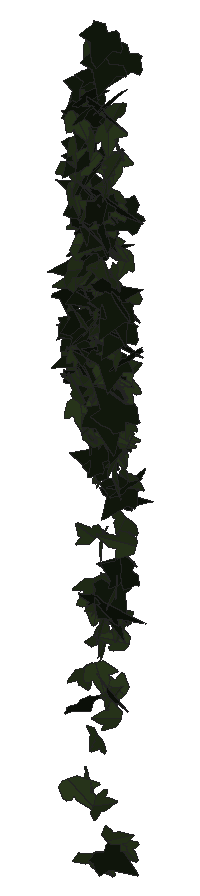
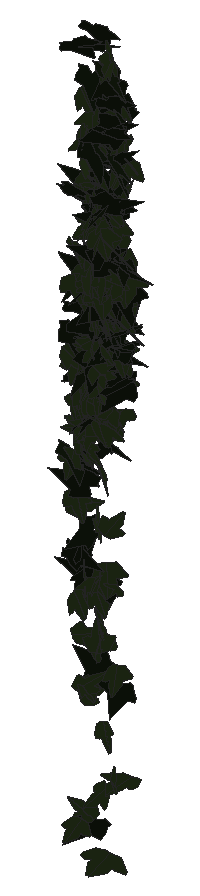
# SketchUp Ruby script. Lengths in millimetres.
U = 1.mm
M = Sketchup.active_model
def pt(a) = Geom::Point3d.new(a.map { |v| v * U })
def face(e, loops, mat)
  f = e.add_face(loops[0].map { |a| pt(a) })
  loops[1..].each { |l| e.add_face(l.map { |a| pt(a) }).erase! }
  f.material = f.back_material = mat if mat
  f
end
# faces: each face lists its corners as indices into pts; further lists are holes
def faces(e, pts, list, mat = nil) = list.each { |f| face(e, (f[0].is_a?(Array) ? f : [f]).map { |l| l.map { |i| pts[i] } }, mat) }
# xy, xz, yz: faces in a plane at the given z, y or x. An outline is a flat list of corners, or four numbers for a rectangle; further outlines are holes
def ring(l) = l.size == 4 ? [[l[0], l[1]], [l[2], l[1]], [l[2], l[3]], [l[0], l[3]]] : l.each_slice(2).to_a
def flat(e, list, mat, &to3) = list.each { |f| face(e, (f[0].is_a?(Array) ? f : [f]).map { |l| ring(l).map { |u, v| to3.(u, v) } }, mat) }
def xy(e, z, list, mat = nil) = flat(e, list, mat) { |x, y| [x, y, z] }
def xz(e, y, list, mat = nil) = flat(e, list, mat) { |x, z| [x, y, z] }
def yz(e, x, list, mat = nil) = flat(e, list, mat) { |y, z| [x, y, z] }
def lines(e, pts, list) = list.each { |a, b| e.add_line(pt(pts[a]), pt(pts[b])) }
# prism: a flat outline (further loops are holes) pulled along v
def prism(e, loops, v, mat = nil)
  f = face(e, loops, mat); d = Geom::Vector3d.new(v.map { |x| x * U })
  f.pushpull(f.normal.samedirection?(d) ? d.length : -d.length)
end
def box(e, o, s, mat = nil) = prism(e, [[o, [o[0] + s[0], o[1], o[2]], [o[0] + s[0], o[1] + s[1], o[2]], [o[0], o[1] + s[1], o[2]]]], [0, 0, s[2]], mat)
def at(x, y, z, deg = 0) = Geom::Transformation.translation(pt([x, y, z])) * Geom::Transformation.rotation(ORIGIN, Z_AXIS, deg.degrees)
def axes(o, x, y, z) = Geom::Transformation.new([*x, 0, *y, 0, *z, 0, *pt(o).to_a, 1])
def part(name) = M.definitions.add(name)
# library, detail: a bought-in or finely detailed component or shape, given as its bounding box
def library(name, o, s) = part(name).tap { |d| box(d.entities, o, s) }
def detail(e, o, s) = box(e.add_group.entities, o, s)
def put(e, d, t, mat = nil) = e.add_instance(d, t).tap { |i| i.material = mat if mat }
def group(e, t, mat = nil) = e.add_group.tap { |g| g.transformation = t; g.material = mat if mat }.entities
root = M.entities
M.materials.add("efeu1").color = [18, 25, 13]
M.materials.add("efeu2").color = [43, 57, 29]
c1 = part("ivyleaf_10")
p = [[0,12.8,-0.8],[-1.5,51.3,-10.9],[-4.9,51,-11.6],[-13.6,26.5,-7.3],[-13.2,15.9,-4.6],[-21.1,19.3,-7.2],
  [-29.5,16.3,-8.3],[-29.2,8.3,-6.2],[-19.7,-9.8,0.5],[-7.6,-13,4],[1,-12.2,5.8],[-0.4,51.1,-11.1],
  [-1.5,51.1,-10.9],[1,-12.4,5.9],[16.9,-12.4,3.5],[35.1,9.1,-5.1],[35,12.9,-6.1],[20.5,16.4,-4.9],
  [15.8,15,-3.8],[15.3,27.6,-7.1],[12.8,31.3,-7.8]]
faces(c1.entities,p,[[0,1,2,3,4,5,6,7,8,9,10],[11,12,0,13,14,15,16,17,18,19,20]],"efeu2")
c2 = part("ivyleaf_9")
p = [[39.1,54.8,31.7],[34.5,51.8,30.2],[-5.3,25.2,17.3],[-17.9,28.3,20.9],[-21.6,21.7,17],[-20.2,4.3,5.3],
  [-22.9,-0.3,2.5],[-17.1,-4,-0.6],[-2,-2.1,-1.2],[-0.7,-15.4,-10.1],[16.6,-22.3,-16.7],[21.1,-15.1,-12.5],
  [32.7,-10.7,-11],[46.1,-1.8,-6.6],[30.8,11.2,3.8]]
faces(c2.entities,p,[[0,1,2,3,4,5,6,7,8,9,10,11,12,13,14]],"efeu1")
put(root,c1,axes([752.7,985.2,1113.9],[-0.74272,0.32931,-0.52967],[-0.59636,0.20777,0.69102],[0.47258,0.77975,0.03957]))
put(root,c2,axes([734.6,998.7,1013.6],[0.71888,0.48535,0.05808],[0.0471,0.04448,-0.76333],[-0.59448,0.59043,0.00976]))
put(root,c1,axes([746.1,992.7,1011.5],[-0.86277,0.0268,-0.17998],[-0.21923,0.01065,0.70769],[0.03488,0.72965,-0.00372]))
put(root,c2,axes([744.8,980.7,1167.3],[0.45026,0.58354,-0.42423],[-0.26636,-0.36384,-0.6904],[-0.8389,0.42872,-0.00848]))
put(root,c2,axes([734.3,1024.5,1017.5],[-0.16118,-0.77907,-0.00625],[-0.00493,0.00702,-0.79017],[0.95048,-0.13207,-0.00516]))
put(root,c1,axes([743.7,985.2,1184.5],[-0.71292,-0.63034,0.00049],[0.00698,-0.00597,-0.8595],[0.76898,-0.58433,0.00825]))
put(root,c2,axes([758.7,1001.5,1208.6],[-0.84853,0.10376,0.4092],[-0.50488,-0.01181,-0.70039],[-0.10172,-0.80687,0.06287]))
put(root,c1,axes([744,999.7,1067.4],[-0.31665,-0.79481,0.09066],[-0.01002,-0.09266,-0.83586],[0.97591,-0.25884,0.02083]))
put(root,c2,axes([746.7,1016.1,1408.8],[-0.72738,0.31029,-0.35451],[0.33499,-0.23579,-0.66816],[-0.46706,-0.65234,0.07288]))
put(root,c1,axes([739,983.2,1341.1],[-0.18555,0.78695,0.1091],[-0.04414,0.1041,-0.80136],[-0.96826,-0.15555,0.01563]))
put(root,c2,axes([758.8,1017.5,1320.6],[-0.28431,0.09191,0.72797],[-0.89505,-0.01646,-0.23278],[-0.01491,-0.76418,0.09257]))
put(root,c1,axes([736,1006.1,962.2],[0.62964,0.64605,0.08333],[0.08075,0.05376,-0.82669],[-0.7906,0.52001,-0.01807]))
put(root,c2,axes([747.1,1019.8,1506.6],[-0.82677,-0.409,-0.01842],[0.01997,0.00852,-0.79154],[0.49909,-0.67788,0.00117]))
put(root,c2,axes([744.2,1009.6,1401.8],[-0.48567,-0.60806,0.27911],[-0.17746,-0.23836,-0.72674],[0.79673,-0.42375,0.00827]))
put(root,c2,axes([751.5,981.2,1221.1],[-0.06903,0.74396,0.27596],[-0.04233,0.27407,-0.746],[-0.96714,-0.06509,0.01296]))
put(root,c2,axes([740.4,1014.4,1457.2],[-0.32635,-0.71367,0.01173],[-0.00513,-0.01096,-0.76215],[0.87078,-0.26753,-0.00009]))
put(root,c2,axes([756.5,1008.3,1060.5],[-0.84556,-0.25006,0.34141],[-0.37588,-0.15097,-0.73603],[0.35394,-0.75772,0.03397]))
put(root,c1,axes([742.2,988.9,1421.9],[0.10068,0.76939,-0.10646],[-0.03631,-0.10384,-0.77358],[-0.9469,0.08579,0.01835]))
put(root,c2,axes([733.9,998.7,1103],[0.03434,-0.77163,-0.17513],[0.21582,0.17695,-0.75118],[0.9409,-0.01242,0.1787]))
put(root,c1,axes([757.1,979.1,994.5],[-0.50932,0.34946,-0.48835],[-0.47788,0.29235,0.54405],[0.5553,0.57211,0.02028]))
put(root,c1,axes([737.1,1002.6,1493.3],[0.76919,-0.31526,0.33383],[0.36271,-0.15187,-0.70491],[0.42691,0.69706,-0.00259]))
put(root,c1,axes([744.1,973.6,1211.4],[-0.12272,-0.31156,-0.81234],[0.23913,0.78861,-0.32673],[1.03416,-0.21932,-0.02084]))
put(root,c1,axes([746.2,1003,509.9],[-0.32891,-0.6822,-0.18443],[0.14876,0.14953,-0.73134],[0.84923,-0.29041,0.05668]))
put(root,c1,axes([745.1,995.2,1064.3],[0.38522,0.78872,-0.0383],[-0.15994,0.01168,-0.84019],[-0.95,0.31786,0.12592]))
put(root,c1,axes([743.1,983.6,1382.8],[-0.93317,-0.27888,-0.30823],[0.36701,0.0741,-0.81355],[0.34996,-0.82133,0.03127]))
put(root,c2,axes([741.9,1028.6,1461.5],[-0.51231,-0.53417,-0.34372],[0.34828,0.20938,-0.67415],[0.69227,-0.50064,0.08479]))
put(root,c1,axes([731.2,1021.7,1194.8],[-0.13541,0.04369,-0.73699],[0.79374,-0.34649,-0.11853],[-0.42575,-0.65987,0.01344]))
put(root,c2,axes([738.2,1002.9,1077.7],[-0.08346,-0.75084,-0.2086],[0.20065,0.19078,-0.74061],[0.9293,-0.10862,0.14118]))
put(root,c2,axes([767.3,983.9,1113.1],[-0.59185,0.61271,0.34592],[-0.42228,0.158,-0.76528],[-0.74737,-0.57449,0.15846]))
put(root,c2,axes([761.8,978.2,1360.9],[-0.21368,0.56186,0.50454],[-0.2383,0.4666,-0.58741],[-0.88993,-0.25986,0.03615]))
put(root,c1,axes([747.1,1019.9,1573.5],[-0.69851,0.54729,-0.1407],[0.13615,-0.08684,-0.79192],[-0.67582,-0.58315,-0.01411]))
put(root,c1,axes([753.3,1003,1280.8],[-0.69561,-0.53486,-0.04718],[0.04265,0.0317,-0.78178],[0.65368,-0.57124,0.0008]))
put(root,c2,axes([759.7,996,1125.2],[0.01509,0.1874,-0.74979],[-0.15022,-0.73983,-0.18694],[-0.93084,0.12243,0.01801]))
put(root,c1,axes([749.5,1002.2,1181.6],[-0.27426,0.70811,0.06754],[-0.02044,0.06554,-0.74293],[-0.86758,-0.22539,-0.00385]))
put(root,c2,axes([740.7,1007.8,1452.2],[0.54896,0.29569,0.54471],[0.49896,0.36412,-0.5355],[-0.56815,0.60548,0.05602]))
put(root,c2,axes([739.3,996.4,1080.8],[1.01247,0.15234,0.10307],[0.10613,0.09458,-0.84026],[-0.19771,0.8309,0.07675]))
put(root,c1,axes([739.1,986.2,318.1],[0.63087,0.54304,0.37357],[0.36941,0.31919,-0.63621],[-1.19883,0.38412,0.00054]))
put(root,c2,axes([768.4,983.2,1410.5],[-0.60889,0.51412,0.30207],[-0.27006,0.20602,-0.71639],[-0.67549,-0.54579,0.01413]))
put(root,c1,axes([754.5,975.5,1365.8],[-0.0166,-0.2923,-0.72557],[0.02877,0.7252,-0.29259],[0.9539,-0.02696,-0.0038]))
put(root,c2,axes([744.2,1003.5,1010.1],[0.94641,0.16518,0.21654],[-0.25875,-0.04369,0.79313],[0.20844,-0.80421,0.00138]))
put(root,c1,axes([740.6,1013.9,323],[0.07057,-0.07394,0.6497],[0.68937,-0.32258,-0.08702],[0.40146,0.56692,0.03522]))
put(root,c1,axes([747.3,982.1,1471.2],[0.38445,0.67535,0.25993],[0.12426,0.23929,-0.7452],[-0.87405,0.33107,0.00839]))
put(root,c1,axes([760.9,1021.8,1170.5],[-0.88189,-0.31484,0.13087],[-0.15821,-0.02985,-0.78808],[0.3847,-0.734,-0.02408]))
put(root,c1,axes([754.8,1013.1,1191.9],[-0.64448,-0.62476,-0.21716],[0.28177,0.16617,-0.70895],[1.22688,-0.36635,0.04875]))
put(root,c2,axes([770,1000.5,1544.9],[-0.43585,0.66482,0.19347],[-0.23195,0.11515,-0.74675],[-0.81225,-0.38962,0.10943]))
put(root,c1,axes([753.7,1029.3,1012.9],[0.29743,-0.59242,0.38429],[0.15919,-0.36175,-0.64046],[0.84666,0.27613,-0.01458]))
put(root,c2,axes([758.5,1007.6,1161],[-0.34037,-0.33499,0.62399],[-0.32097,-0.57365,-0.4256],[0.80221,-0.37166,0.09447]))
put(root,c1,axes([762.8,1000.9,748.6],[-0.38117,-0.36304,-0.47507],[-0.3995,-0.34459,0.47868],[-0.61033,0.45229,-0.01663]))
put(root,c1,axes([762.3,1020.2,1267.8],[-0.62513,-0.51644,0.16325],[-0.13419,-0.12083,-0.72747],[0.64701,-0.52403,0.00685]))
put(root,c1,axes([766.8,1007.7,1306.9],[-0.5087,-0.3947,0.51197],[-0.37991,-0.41126,-0.57067],[0.69114,-0.51657,0.06314]))
put(root,c2,axes([758,975.2,469.8],[0.33013,0.7053,0.15299],[0.05785,0.14566,-0.75539],[-0.87857,0.27461,0.00775]))
put(root,c2,axes([764.4,985.2,1106.3],[-0.09778,0.77152,0.09421],[0.00785,0.09537,-0.7755],[-0.94821,-0.07877,-0.01613]))
put(root,c1,axes([759.1,1022.6,1130.9],[0.53282,-0.67818,0.01963],[-0.00184,-0.02164,-0.73363],[1.29125,0.27981,-0.00914]))
put(root,c2,axes([753.5,1012.5,1224.1],[0.56312,0.47025,0.48001],[-0.48839,-0.2753,0.65464],[0.65845,-0.60636,0.07504]))
put(root,c2,axes([770.6,979.7,1489.3],[-0.30189,0.70178,0.28483],[-0.17064,0.25215,-0.74277],[-0.90811,-0.28068,0.04488]))
put(root,c2,axes([750.5,1001.8,1340.9],[0.80382,-0.48789,-0.17009],[0.16692,-0.10105,0.81984],[-0.60785,-0.67292,0.0002]))
put(root,c2,axes([753.8,1005.7,1309.2],[-0.36235,-0.75287,-0.19878],[0.09325,0.18354,-0.80933],[0.94538,-0.30667,0.00364]))
put(root,c1,axes([765.7,1021,1030.6],[-0.37697,-0.53893,0.41581],[-0.09369,-0.42058,-0.56856],[1.2921,-0.18773,0.08009]))
put(root,c1,axes([744.8,1016.6,1578.4],[0.47366,-0.24458,0.67301],[0.76149,-0.25963,-0.45442],[0.42818,0.7323,0.06367]))
put(root,c2,axes([747,997.4,1048.3],[0.99421,0.12743,-0.00059],[-0.00077,0.0079,0.82479],[0.15546,-0.81489,0.0079]))
put(root,c1,axes([761.1,1006.5,1139.6],[0.68466,-0.46532,-0.04269],[-0.03906,0.02827,-0.72901],[0.56873,0.56211,0.00133]))
put(root,c1,axes([770.8,1002.7,403.6],[-0.69414,0.22339,0.37456],[-0.46695,0.03937,-0.60488],[-0.25505,-0.68005,0.08802]))
put(root,c1,axes([744.2,1001.6,934.3],[-0.10581,0.07527,-0.73247],[0.70018,-0.63346,-0.09302],[-1.21393,-0.37193,0.01019]))
put(root,c1,axes([751.1,1019.5,970.7],[-0.74451,-0.10632,-0.51653],[0.64334,-0.13209,-0.59582],[-0.00739,-0.78852,0.16945]))
put(root,c1,axes([753.2,1028,1082.7],[0.86494,-0.46224,0.32748],[0.46577,-0.21843,-0.64796],[0.97235,0.51582,0.01908]))
put(root,c2,axes([778.3,1007.9,1260.7],[-1.24453,0.36445,-0.12591],[0.19682,-0.07305,-0.7485],[-0.70697,-0.66191,0.01327]))
put(root,c1,axes([757,1014.7,189.4],[-1.09388,-0.29866,-0.31656],[0.51916,0.16139,-0.64753],[0.6454,-0.63601,-0.01566]))
put(root,c1,axes([761.2,1024.4,559.9],[-0.35956,-0.72736,-0.06906],[-0.03216,-0.06383,0.7848],[-0.89079,0.2959,-0.00046]))
put(root,c1,axes([767.3,999.9,946.7],[0.07261,-0.66931,-0.19407],[-0.06564,0.19231,-0.67002],[1.32468,0.04622,-0.02256]))
put(root,c1,axes([763.9,1017.1,1002.5],[-0.27661,-0.71632,-0.2254],[0.10368,0.20946,-0.75115],[0.91027,-0.24153,0.01706]))
put(root,c1,axes([752.4,983.7,1253.7],[-0.22029,-0.24308,-0.707],[0.65675,0.46244,-0.29648],[0.63293,-0.56445,0.06157]))
put(root,c1,axes([766.6,992,1082.3],[0.68433,-0.54131,-0.25315],[-0.19851,0.19574,-0.77907],[0.7015,0.58345,0.0265]))
put(root,c1,axes([759.5,1021.3,936.9],[1.30927,-0.08791,0.00717],[0.01336,-0.00165,-0.69353],[0.16733,0.68797,-0.00075]))
put(root,c1,axes([770.6,1007.6,1205.5],[0.14216,0.36173,-0.6354],[-0.46716,-0.51793,-0.36507],[-0.75989,0.38608,0.10557]))
put(root,c1,axes([769.6,1011.7,859.3],[0.53758,-0.60836,-0.27966],[-0.1588,0.26918,-0.66983],[1.26437,0.29247,0.03477]))
put(root,c1,axes([772.1,986.5,1439.2],[0.4867,-0.43032,-0.51826],[-0.35701,0.43181,-0.5838],[0.74022,0.4912,0.05918]))
put(root,c1,axes([771.2,994.4,1402.9],[0.78137,0.16565,-0.40422],[-0.47439,-0.11073,-0.66149],[-0.24288,0.74922,-0.00839]))
put(root,c2,axes([748.8,989.4,1465.4],[-0.02768,-0.17555,0.78499],[0.97498,-0.09423,0.00203],[0.11161,0.77965,0.17699]))
put(root,c2,axes([750.3,1010.5,1228.4],[0.36452,0.58881,-0.48771],[0.27693,0.4317,0.66025],[0.8907,-0.37518,-0.00569]))
put(root,c1,axes([769.9,998.1,1122.5],[0.11673,-0.68795,-0.34016],[0.0039,0.34139,-0.69007],[1.46061,0.05407,0.02903]))
put(root,c1,axes([770.4,996,674.7],[-0.52141,-0.72903,-0.05451],[0.02024,0.05346,-0.84497],[0.89167,-0.42752,-0.0127]))
put(root,c1,axes([775.3,1022.7,978.2],[-0.47963,-0.56195,0.30563],[-0.20404,-0.25597,-0.68576],[0.75328,-0.42714,0.00885]))
put(root,c1,axes([780.6,1012.5,1046.7],[-0.11907,-0.13301,0.70046],[-0.53382,-0.54702,-0.16484],[0.68676,-0.44826,-0.00668]))
put(root,c1,axes([769.7,1017.2,1258.4],[-0.41986,0.61957,0.16459],[-0.12069,0.13325,-0.70842],[-0.77273,-0.35745,0.02121]))
put(root,c1,axes([777.8,1012.8,1157.6],[0.4624,0.21791,-0.56361],[-0.59716,-0.2794,-0.43719],[-0.43228,0.61906,0.00107]))
put(root,c2,axes([763,1007.7,1320],[0.7022,-0.35458,-0.36575],[-0.35919,0.21882,-0.67544],[0.50717,0.64589,0.02804]))
put(root,c2,axes([759.4,1006.8,1331.3],[-0.33075,-0.32834,-0.63014],[0.52362,0.46183,-0.4253],[0.69085,-0.50723,0.02066]))
put(root,c1,axes([760.8,1028.2,551.4],[-0.125,0.01438,0.77216],[0.58035,-0.61244,0.07452],[0.74224,0.48129,0.07177]))
put(root,c1,axes([768.1,1009.7,991.1],[0.67955,-0.56386,0.22717],[0.21763,-0.19645,-0.66735],[1.13629,0.37484,-0.00804]))
put(root,c1,axes([772.1,1028.5,977.1],[0.01668,-0.42646,0.5977],[0.08647,-0.59424,-0.42562],[0.89159,0.06561,0.0301]))
put(root,c1,axes([768,1020.2,667.8],[-0.19647,0.54448,-0.30768],[0.08802,-0.29943,-0.56763],[-0.7579,-0.17592,0.01384]))
put(root,c2,axes([769.4,970.8,1514.6],[0.40436,0.50901,0.52105],[0.26186,0.47879,-0.60426],[-0.8492,0.39001,0.06177]))
put(root,c2,axes([790.9,986.3,891.5],[-0.57305,0.32639,0.50895],[-0.50673,0.29414,-0.57197],[-0.53602,-0.627,-0.00339]))
put(root,c2,axes([755.2,986,1280],[0.46728,0.07637,0.71638],[0.86172,0.12,-0.39043],[-0.17312,0.80343,-0.00978]))
put(root,c1,axes([773.3,1013.5,604],[0.4565,-0.72575,0.07772],[0.07501,-0.05569,-0.81601],[0.88731,0.37809,0.02899]))
put(root,c2,axes([762.9,999.1,1142],[0.85383,0.25095,0.17026],[0.19347,0.06216,-0.74347],[-0.31535,0.71758,0.00486]))
put(root,c2,axes([758,986.8,1284.9],[0.8151,-0.36657,0.18485],[0.19346,-0.09525,-0.76204],[0.46199,0.68664,-0.00702]))
put(root,c1,axes([774,1012.4,990.2],[-0.54849,0.58765,0.02322],[-0.01822,0.01781,-0.7399],[-0.71726,-0.44983,0.00104]))
put(root,c1,axes([760.9,1005.3,1110.4],[0.64808,0.17237,0.52143],[0.57629,0.2266,-0.55615],[-0.34173,0.70903,0.05098]))
put(root,c2,axes([776.1,1007.3,1046.4],[0.4753,0.68385,-0.04177],[-0.03789,-0.03037,-0.78695],[-0.83499,0.39065,0.01194]))
put(root,c1,axes([771.9,1000.1,645.1],[0.89376,0.3693,-0.03012],[-0.03127,-0.01606,-0.8204],[-0.45096,0.73303,-0.0028]))
put(root,c1,axes([772.6,1006,1051.9],[0.8126,0.36568,-0.02318],[-0.03403,0.00266,-0.75968],[-0.44572,0.66646,0.01575]))
put(root,c1,axes([780.4,1006.5,637.5],[-0.18943,-0.79477,0.13566],[-0.06638,-0.12751,-0.80929],[0.9814,-0.16203,-0.02856]))
put(root,c1,axes([777.5,981.5,1326.8],[-0.1783,-0.59855,-0.50014],[0.12044,0.49056,-0.61592],[0.94395,-0.17565,-0.01589]))
put(root,c1,axes([774,1000.3,291.4],[-0.10949,-0.24113,-0.73636],[0.28933,0.69716,-0.25719],[0.89993,-0.25347,-0.0069]))
put(root,c1,axes([779,1030.8,919.1],[-0.05833,0.27412,-0.61443],[-0.17643,-0.60577,-0.259],[-0.80164,0.11338,0.10171]))
put(root,c1,axes([773.1,1011.7,1066.8],[-0.60652,-0.34902,-0.37461],[0.41908,0.15982,-0.60478],[0.46319,-0.60162,0.05667]))
put(root,c2,axes([796.5,993,1323.1],[-0.24226,0.26734,0.70436],[-0.63471,0.47819,-0.32817],[-0.6648,-0.55398,0.05664]))
put(root,c1,axes([788.1,1003.5,1019.5],[-0.84528,-0.05354,0.28431],[-0.34312,-0.0483,-0.69449],[0.08273,-0.74736,0.02452]))
put(root,c1,axes([774.4,1033.6,1176.5],[0.01711,-0.49345,-0.52699],[0.10158,-0.52246,0.49143],[-0.87489,-0.07031,0.04675]))
put(root,c2,axes([788.7,1004.6,871.5],[-0.58975,-0.58149,0.19912],[0.16869,0.14395,0.75606],[-0.73064,0.5026,0.01383]))
put(root,c2,axes([769.5,1019.2,952.1],[0.25442,-0.66223,-0.3633],[-0.00599,0.3757,-0.68764],[0.92149,0.18528,0.09584]))
put(root,c1,axes([776.4,1003.5,1023.9],[0.66276,-0.60547,0.27751],[0.26473,-0.24013,-0.69847],[1.23966,0.37499,0.00079]))
put(root,c2,axes([783.5,1005.4,1411.5],[-0.69922,0.13169,-0.49289],[0.50498,-0.31333,-0.56503],[-0.36386,-0.68793,0.163]))
put(root,c1,axes([779.9,1005.4,1329],[0.05663,-0.58409,0.4608],[0.21368,-0.44014,-0.57555],[0.88214,0.14411,0.10983]))
put(root,c1,axes([785.6,1002,1120.9],[-0.14296,-0.70973,-0.23758],[0.07901,0.23446,-0.71352],[1.42224,-0.08436,0.01575]))
put(root,c1,axes([779,1015.8,660.8],[0.19852,0.7537,0.11512],[0.03005,0.11246,-0.77107],[-0.92969,0.16458,-0.00034]))
put(root,c1,axes([790.7,1028.7,479.6],[0.21491,0.46603,0.56658],[-0.31958,-0.50431,0.49626],[0.83601,-0.31258,0.04406]))
put(root,c2,axes([792.2,1002.9,1404.9],[-0.12534,0.75967,-0.0663],[-0.00942,-0.06794,-0.7664],[-0.93027,-0.10167,0.01669]))
put(root,c1,axes([785.2,1016.7,963.4],[-0.03551,-0.29855,0.61547],[0.05508,-0.61552,-0.29644],[0.83273,0.02798,0.04586]))
put(root,c2,axes([786.4,1005.9,1615.3],[-0.8583,-0.30417,-0.2809],[0.31448,0.11162,-0.76646],[0.39529,-0.74926,-0.00015]))
put(root,c1,axes([795.4,994.1,1297.8],[0.69978,-0.02819,-0.53938],[-0.65169,0.08681,-0.57259],[0.0975,0.78256,0.04409]))
put(root,c1,axes([802.8,1017.9,1174.6],[-0.91174,0.36937,-0.43856],[-0.68094,0.25401,0.60476],[0.85274,0.59775,0.01401]))
put(root,c1,axes([793.3,1023.7,893.9],[0.69296,-0.05209,-0.42582],[-0.51666,0.04478,-0.57037],[0.0836,0.70848,0.00474]))
put(root,c2,axes([795.7,996.5,1288.8],[-0.93874,-0.09746,0.02751],[-0.03325,-0.00375,-0.77561],[0.11899,-0.76994,0.0003]))
put(root,c1,axes([781.1,1011,1169.4],[0.37611,0.63854,0.09708],[0.04979,0.08809,-0.70906],[-0.78639,0.31097,0.00154]))
put(root,c1,axes([777.4,1005.9,740.5],[0.20934,-0.46643,-0.6223],[0.25704,-0.58556,0.49698],[-0.91331,-0.27171,-0.00277]))
put(root,c1,axes([797.7,1028.4,567.4],[0.10755,0.13501,0.65877],[-0.53618,-0.49131,0.1595],[0.62095,-0.44763,0.02363]))
put(root,c2,axes([774.2,995.8,1048.4],[0.59658,-0.5648,-0.40158],[-0.29022,0.37374,-0.64467],[1.28662,0.34619,0.04079]))
put(root,c1,axes([804,1008,1145.2],[-0.30213,0.06834,0.70542],[-0.86456,-0.01368,-0.24746],[-0.0118,-0.7475,0.06903]))
put(root,c2,axes([781,1005.7,1295.4],[-0.56599,-0.15637,-0.58102],[0.67719,0.17195,-0.48948],[0.28333,-0.72336,0.00925]))
put(root,c1,axes([791,1021.6,482.6],[-0.1179,-0.61475,0.18438],[0.03604,-0.18691,-0.61681],[1.22095,-0.05385,0.03601]))
put(root,c1,axes([785.2,1021.6,1002.9],[-0.37094,0.60529,-0.18977],[0.10311,-0.16991,-0.67736],[-0.76699,-0.31558,0.00071]))
put(root,c1,axes([792.6,1003.3,1348.5],[-0.94032,-0.02347,0.01456],[-0.01762,-0.00393,-0.7711],[0.02872,-0.77088,0.00349]))
put(root,c1,axes([780.4,1015.4,1063.6],[0.13496,-0.1787,0.75635],[0.61599,-0.56425,-0.20716],[0.72079,0.51567,0.03543]))
put(root,c2,axes([773.9,984.7,1501.2],[0.8422,-0.30203,0.29474],[0.33066,-0.11584,-0.7535],[0.39463,0.74162,0.00234]))
put(root,c1,axes([783.7,1003.4,1046.6],[0.52905,0.38238,0.48901],[0.25593,0.47114,-0.55444],[-0.71277,0.45299,0.16388]))
put(root,c1,axes([795,991,1029],[-0.75374,-0.48272,-0.06297],[0.06251,0.03671,-0.78403],[0.5906,-0.61993,0.00261]))
put(root,c1,axes([786.5,982.4,536],[0.53177,0.56842,0.17247],[0.12704,0.13749,-0.71631],[-0.71347,0.44815,0.001]))
put(root,c2,axes([792.5,974.2,1316.8],[-0.17715,-0.29097,0.75939],[0.58485,0.59249,0.31869],[-0.80142,0.4967,0.06471]))
put(root,c2,axes([798.9,997.3,1037.9],[0.59109,0.4582,-0.40223],[-0.43211,-0.20667,-0.66206],[-0.60546,0.59483,0.07981]))
put(root,c1,axes([780.1,1015.1,1149],[0.54503,-0.00697,0.55607],[0.67831,-0.00955,-0.4468],[0.01441,0.71323,-0.00055]))
put(root,c1,axes([796.2,1016.2,887.5],[0.21536,-0.6648,0.12809],[0.09183,-0.12162,-0.67383],[1.28524,0.12009,0.02668]))
put(root,c1,axes([794.3,1018.8,986],[-0.19228,0.51742,-0.47375],[-0.12882,-0.48359,-0.51374],[-1.32895,-0.02799,0.11834]))
put(root,c1,axes([769,997.8,925.4],[-0.12463,-0.03632,-0.74246],[1.40457,0.08607,-0.0693],[0.16941,-0.74036,0.02836]))
put(root,c1,axes([798.3,991.6,1204.6],[-0.92662,0.14608,0.00324],[-0.00276,-0.02889,0.77291],[0.17824,0.75899,0.0288]))
put(root,c2,axes([782.9,1015.8,748.3],[0.86161,-0.29216,-0.01882],[-0.02006,0.00948,-0.76428],[0.35661,0.70642,0.00247]))
put(root,c1,axes([786.8,1005.3,1296.7],[-0.58979,0.19234,-0.52331],[0.46148,-0.3957,-0.49487],[-0.49971,-0.59244,0.16064]))
put(root,c1,axes([804,1005.5,1327.9],[0.77006,-0.02327,-0.4378],[-0.53082,0.06103,-0.63055],[0.06571,0.76574,0.03695]))
put(root,c1,axes([788.3,1015.7,929.3],[0.42796,0.51922,0.37715],[0.25949,0.31146,-0.62661],[-0.73868,0.41023,-0.00162]))
put(root,c2,axes([795.2,1003.8,1031.1],[0.83927,-0.00064,-0.44396],[-0.52349,0.20912,-0.6652],[0.13897,0.79159,0.17537]))
put(root,c1,axes([792.6,985.9,1071.3],[-0.7751,-0.28347,-0.34153],[0.42004,0.06158,-0.6916],[0.34172,-0.71868,0.07545]))
put(root,c2,axes([786.4,1006.9,638.6],[0.38841,-0.74494,-0.13559],[-0.0204,0.14013,-0.80918],[0.92354,0.31639,0.03915]))
put(root,c1,axes([795.3,998.4,1457],[0.38988,0.70205,-0.07493],[-0.05491,-0.06182,-0.77121],[-0.85962,0.32236,0.01528]))
put(root,c2,axes([794.7,999.6,1575.9],[-0.54657,-0.6677,-0.02671],[0.2675,-0.1165,-0.76525],[0.77012,-0.43342,0.24685]))
put(root,c2,axes([794.4,987.2,1295.3],[0.66505,-0.39287,-0.54286],[-0.5103,0.34724,-0.67132],[0.63871,0.6865,0.0289]))
put(root,c1,axes([801.9,1011.2,1430.9],[-0.6018,0.55088,0.22236],[-0.18085,0.16573,-0.73945],[-0.70183,-0.51507,-0.00012]))
put(root,c1,axes([797.8,999.8,1277.3],[-0.2914,0.72018,0.10211],[-0.03741,0.09741,-0.75875],[-0.88662,-0.24081,-0.00154]))
put(root,c1,axes([803.9,1002.9,449.1],[0.04471,0.20392,0.67379],[-0.13036,-0.66527,0.20716],[0.84889,-0.1129,-0.00368]))
put(root,c1,axes([802.4,1002.9,1375.3],[0.0146,-0.75781,0.18894],[0.05714,-0.18852,-0.75736],[1.48532,0.0147,0.02728]))
put(root,c2,axes([807.5,985.9,1515.2],[-0.04209,0.77818,0.12393],[-0.02995,0.12292,-0.77872],[-0.96088,-0.03792,0.01884]))
put(root,c1,axes([804.5,1002.7,670.3],[0.19094,-0.64294,-0.52047],[-0.13081,0.50947,-0.66159],[1.00067,0.18928,0.01283]))
put(root,c2,axes([778.9,1000.8,500.3],[0.39209,-0.41465,0.62014],[0.45295,-0.57321,-0.46233],[1.34559,0.31377,-0.02507]))
put(root,c2,axes([793,1006.3,671.5],[0.10378,-0.69083,-0.44087],[-0.04249,0.43979,-0.69586],[0.99891,0.09048,0.0162]))
put(root,c1,axes([791.1,995,1265.8],[-0.70695,-0.09583,-0.54206],[0.65121,0.09451,-0.58732],[0.16411,-0.78783,-0.00451]))
put(root,c2,axes([783.2,999.6,1102.9],[0.90193,-0.09917,0.34207],[0.41376,-0.04465,-0.74591],[0.13269,0.81337,0.00076]))
put(root,c1,axes([789,1011.5,1023.6],[0.0295,-0.23651,-0.6799],[0.53864,-0.53244,0.20091],[-0.69366,-0.42351,0.1271]))
put(root,c1,axes([801.7,983.5,1376.8],[0.53144,-0.6487,-0.33393],[0.11849,0.37743,-0.68115],[1.38352,0.21686,0.18661]))
put(root,c2,axes([803.5,1015,691.9],[-0.00404,0.10101,0.758],[-0.47534,-0.65246,0.08525],[0.80275,-0.38584,0.05429]))
put(root,c1,axes([805.1,1007.9,1493.2],[-0.13991,-0.73234,0.25084],[-0.01236,-0.25213,-0.74076],[0.94433,-0.11181,0.02747]))
put(root,c1,axes([796.2,1012.3,913],[-0.66236,0.2703,-0.30513],[0.33768,-0.12863,-0.60644],[-0.36509,-0.60936,-0.00734]))
put(root,c1,axes([805,1016.3,980.5],[-0.0529,-0.79501,-0.09733],[-0.00215,0.09757,-0.79616],[0.97715,-0.04282,-0.00702]))
put(root,c2,axes([821.4,1018.5,702.4],[-0.28077,0.01953,-0.72477],[-0.78845,-0.35021,0.19577],[-0.40096,0.67499,0.12254]))
put(root,c1,axes([787.7,1013.2,924.7],[-0.13328,-0.09476,-0.73448],[0.84308,0.25389,-0.13554],[0.32485,-0.69781,0.05043]))
put(root,c1,axes([794.1,991.5,1055.1],[0.32726,0.56099,0.52859],[0.29161,0.47156,-0.62176],[-0.89401,0.35917,-0.00931]))
put(root,c2,axes([799,1019.5,931],[-0.16281,-0.72679,0.29694],[-0.05059,-0.29425,-0.73885],[0.9565,-0.13928,0.01146]))
put(root,c2,axes([797,991.1,974.6],[-0.4647,-0.56241,-0.48282],[0.43017,0.34001,-0.67422],[0.79544,-0.51244,0.08255]))
put(root,c2,axes([778.3,1002.1,1331.7],[0.4441,-0.40053,0.61952],[0.87701,-0.42829,-0.45045],[1.09643,0.50481,0.10937]))
put(root,c1,axes([811.5,1018.1,1172],[-0.83945,-0.58454,0.14421],[0.02068,-0.18646,-0.7226],[1.14567,-0.42494,0.1187]))
put(root,c2,axes([774.7,987,642],[1.0169,0.13221,-0.57329],[1.0409,0.17381,0.54982],[0.41269,-0.76416,0.02587]))
put(root,c1,axes([814.9,1002.1,1054.3],[0.50564,0.38314,-0.61383],[-0.69373,-0.494,-0.46611],[-1.18964,0.45092,0.01091]))
put(root,c1,axes([804.8,1002.4,1410.3],[0.37233,0.6869,-0.11948],[-0.06489,-0.1071,-0.75163],[-0.84812,0.30974,0.00506]))
put(root,c1,axes([811.9,1015.3,621],[-0.18736,-0.74557,0.25804],[0.06986,-0.27272,-0.75392],[0.96,-0.12567,0.10523]))
put(root,c2,axes([800.9,1008.5,1154.2],[0.20686,-0.80811,-0.09241],[-0.03264,0.08881,-0.82567],[0.99178,0.17148,-0.0079]))
put(root,c1,axes([820.9,1008,791.3],[-0.83722,0.01569,0.35719],[-0.43615,-0.04105,-0.68504],[0.00617,-0.77255,0.04366]))
put(root,c1,axes([810,1022,1235.2],[0.82872,-0.29894,-0.04096],[-0.04392,0.01989,-0.74214],[0.36549,0.68023,0.0037]))
put(root,c2,axes([792.3,999.1,1175.6],[0.1394,-0.18914,0.75301],[0.91454,-0.1713,-0.15677],[0.24662,0.74212,0.15573]))
put(root,c1,axes([815.1,991.8,1087.2],[0.7444,-0.6209,-0.24164],[-0.14831,0.23565,-0.73164],[1.25934,0.39477,0.05667]))
put(root,c2,axes([802.2,985.1,223.4],[0.04234,-0.19447,-0.75689],[0.07084,0.75618,-0.19163],[0.95076,-0.04768,0.04798]))
put(root,c2,axes([805.2,998.1,1073.5],[-0.34917,-0.78529,0.08726],[0.19846,-0.14939,-0.81083],[0.9433,-0.25925,0.20289]))
put(root,c2,axes([815.4,1019.6,1583.8],[-0.68248,-0.57491,0.05908],[-0.06588,-0.02987,-0.80196],[0.702,-0.56172,-0.01783]))
put(root,c1,axes([814.2,995.9,1415.7],[0.06885,-0.71724,0.38027],[0.02879,-0.37958,-0.71944],[0.98999,0.06092,-0.00553]))
put(root,c2,axes([816.4,1008.2,1125.5],[-0.77406,-0.50927,-0.0238],[0.0253,0.01218,-0.81357],[0.62147,-0.6348,0.00348]))
put(root,c1,axes([801,1005,1209.6],[-0.06777,0.12773,-0.75309],[0.49137,-0.63668,-0.13769],[-0.79181,-0.40603,-0.02099]))
put(root,c2,axes([815.6,999.2,1165.2],[-0.72747,-0.57435,-0.02227],[0.01622,0.0183,-0.82791],[0.70105,-0.59642,-0.00395]))
put(root,c1,axes([819.5,1027.1,1048.5],[-0.17506,-0.59474,0.39006],[-0.08967,-0.38735,-0.60172],[1.35067,-0.1028,0.01061]))
put(root,c1,axes([810,1014.5,1019.3],[-0.91349,-0.05012,-0.27636],[0.33552,-0.29066,-0.6924],[-0.0696,-0.74333,0.28938]))
put(root,c1,axes([802.5,999.1,240.9],[-0.46698,-0.1538,0.55478],[0.62588,0.2112,0.4125],[-0.31873,0.64007,-0.00281]))
put(root,c1,axes([822.9,981.7,871.8],[-0.46557,0.42829,0.59903],[-0.49739,0.43897,-0.57358],[-0.74815,-0.55837,0.00855]))
put(root,c1,axes([809.1,1019.1,959.1],[0.92398,-0.19991,0.11823],[0.16881,0.0645,-0.77732],[0.22758,0.76381,0.09659]))
put(root,c2,axes([795.2,1012.7,819.2],[0.33574,-0.14159,0.70585],[0.85055,-0.13602,-0.2991],[0.21901,0.74529,0.0795]))
put(root,c2,axes([821.2,1008.3,846],[-0.90766,-0.2327,-0.09939],[0.11634,0.02806,-0.77953],[0.28595,-0.75007,0.00167]))
put(root,c1,axes([814.8,1025,923.1],[0.55022,-0.63741,0.13207],[0.10902,-0.11904,-0.6999],[1.23408,0.29471,0.00294]))
put(root,c2,axes([809.1,998.4,1177.9],[0.98981,-0.2853,-0.47806],[-0.69697,0.31744,-0.58783],[0.79806,0.63108,0.07956]))
put(root,c1,axes([816.6,1010.2,969.5],[0.13909,-0.7578,0.17561],[0.06136,-0.16994,-0.76596],[0.94703,0.12231,0.02383]))
put(root,c1,axes([812.5,1012.1,227],[-0.47947,-0.40252,-0.36821],[0.35045,0.23311,-0.56143],[0.56581,-0.48549,0.03571]))
put(root,c2,axes([831.2,1000,856.6],[-0.02377,0.75894,0.37765],[-0.27755,0.35921,-0.73362],[-0.99626,-0.11818,0.19537]))
put(root,c2,axes([834.9,986,978.4],[-0.97673,-0.56091,0.15021],[0.22725,0.09425,0.75988],[-1.08152,0.52636,0.02401]))
put(root,c1,axes([822.5,1016.6,863.6],[-0.86087,0.24489,0.03144],[-0.03703,0.00844,-0.74692],[-0.29894,-0.70628,0.00198]))
put(root,c2,axes([828.9,1001.4,1075.9],[-0.14447,0.79962,-0.14954],[0.03652,-0.14673,-0.8083],[-0.99177,-0.12188,-0.00798]))
put(root,c2,axes([834.8,1011.1,1322.6],[-0.97086,0.02715,0.13407],[-0.16388,-0.00566,-0.79619],[-0.03151,-0.80698,0.0101]))
put(root,c1,axes([838.6,992.2,764.4],[-0.18811,-0.03304,-0.78548],[-0.91665,-0.2294,0.15714],[-0.2823,0.7669,0.01316]))
put(root,c1,axes([826.2,1000.2,978.5],[0.50002,-0.53473,-0.38107],[-0.14211,0.38345,-0.58955],[1.24157,0.25924,0.08599]))
